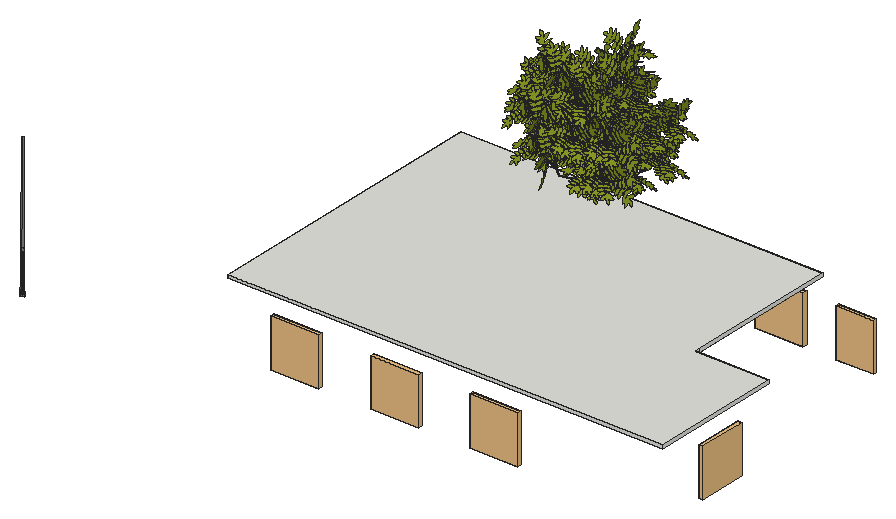
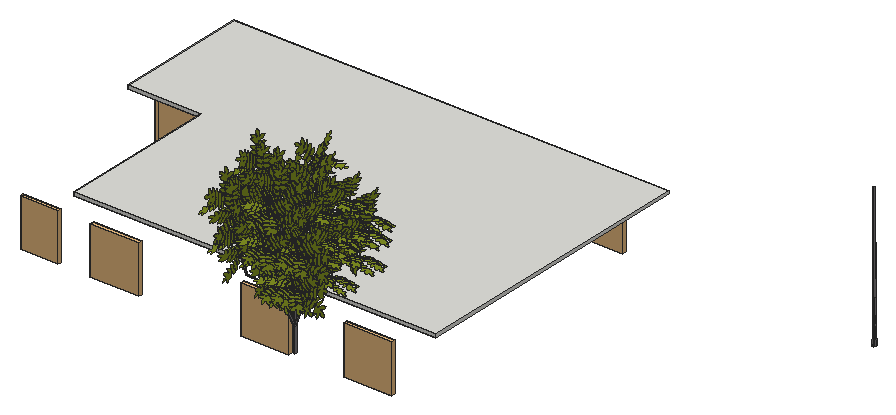
# SketchUp Ruby script. Lengths in inches.
U = 1.inch
M = Sketchup.active_model
def pt(a) = Geom::Point3d.new(a.map { |v| v * U })
def face(e, loops, mat)
  f = e.add_face(loops[0].map { |a| pt(a) })
  loops[1..].each { |l| e.add_face(l.map { |a| pt(a) }).erase! }
  f.material = f.back_material = mat if mat
  f
end
# faces: each face lists its corners as indices into pts; further lists are holes
def faces(e, pts, list, mat = nil) = list.each { |f| face(e, (f[0].is_a?(Array) ? f : [f]).map { |l| l.map { |i| pts[i] } }, mat) }
# xy, xz, yz: faces in a plane at the given z, y or x. An outline is a flat list of corners, or four numbers for a rectangle; further outlines are holes
def ring(l) = l.size == 4 ? [[l[0], l[1]], [l[2], l[1]], [l[2], l[3]], [l[0], l[3]]] : l.each_slice(2).to_a
def flat(e, list, mat, &to3) = list.each { |f| face(e, (f[0].is_a?(Array) ? f : [f]).map { |l| ring(l).map { |u, v| to3.(u, v) } }, mat) }
def xy(e, z, list, mat = nil) = flat(e, list, mat) { |x, y| [x, y, z] }
def xz(e, y, list, mat = nil) = flat(e, list, mat) { |x, z| [x, y, z] }
def yz(e, x, list, mat = nil) = flat(e, list, mat) { |y, z| [x, y, z] }
def lines(e, pts, list) = list.each { |a, b| e.add_line(pt(pts[a]), pt(pts[b])) }
# prism: a flat outline (further loops are holes) pulled along v
def prism(e, loops, v, mat = nil)
  f = face(e, loops, mat); d = Geom::Vector3d.new(v.map { |x| x * U })
  f.pushpull(f.normal.samedirection?(d) ? d.length : -d.length)
end
def box(e, o, s, mat = nil) = prism(e, [[o, [o[0] + s[0], o[1], o[2]], [o[0] + s[0], o[1] + s[1], o[2]], [o[0], o[1] + s[1], o[2]]]], [0, 0, s[2]], mat)
def at(x, y, z, deg = 0) = Geom::Transformation.translation(pt([x, y, z])) * Geom::Transformation.rotation(ORIGIN, Z_AXIS, deg.degrees)
def axes(o, x, y, z) = Geom::Transformation.new([*x, 0, *y, 0, *z, 0, *pt(o).to_a, 1])
def part(name) = M.definitions.add(name)
# library, detail: a bought-in or finely detailed component or shape, given as its bounding box
def library(name, o, s) = part(name).tap { |d| box(d.entities, o, s) }
def detail(e, o, s) = box(e.add_group.entities, o, s)
def put(e, d, t, mat = nil) = e.add_instance(d, t).tap { |i| i.material = mat if mat }
def group(e, t, mat = nil) = e.add_group.tap { |g| g.transformation = t; g.material = mat if mat }.entities
root = M.entities
M.materials.add("3D66_SU_1574822641685_001").color = [135, 150, 36]
M.materials.add("3D66_SU_1574822641883_002").color = [178, 165, 164]
M.materials.add("3D66_SU_1574822642012_003").color = [128, 125, 127]
c1 = library("4e1fe49e-2fec-46be-a265-c81cc17eb477",[0,0,0],[35.43,4.93,59.06])
c2 = part("rama-acacia")
p = [[-13.8,1.01,-1.08],[-13.61,0.91,-1.04],[-13.61,0.85,-1.06],[-14.07,0.85,-1.21],[-15.17,0.86,-1.58],[-15.95,0.92,-1.83],
  [-16.01,1,-1.83],[-16.01,1.17,-1.78],[-16.07,1.93,-1.6],[-16.4,2.73,-1.5],[-16.65,3.06,-1.5],[-17.13,4.01,-1.41],
  [-17.78,4.7,-1.44],[-18.28,5.07,-1.51],[-18.57,5.18,-1.58],[-18.91,5.47,-1.62],[-19.07,5.48,-1.67],[-19.35,5.61,-1.73],
  [-19.51,5.64,-1.78],[-19.38,5.57,-1.75],[-19.33,5.5,-1.75],[-19.31,5.23,-1.82],[-19.38,5.08,-1.89],[-19.41,4.84,-1.96],
  [-19.36,4.59,-2.01],[-19.43,4.55,-2.04],[-19.36,4.15,-2.125],[-19.21,3.7,-2.19],[-18.875,3.1,-2.24],[-18.61,2.78,-2.24],
  [-17.83,2.19,-2.13],[-17.4375,1.85,-2.09],[-17.04,1.49,-2.05],[-16.61,1.24,-1.97],[-16.17,1.0625,-1.87],[-16.06,0.95,-1.86],
  [-16.06,0.91,-1.87],[-16.32,0.9,-1.96],[-16.7,0.88,-2.1],[-17.05,0.91,-2.21],[-17.61,1.15,-2.33],[-18.06,1.29,-2.45],
  [-18.88,1.53,-2.67],[-20.25,1.46,-3.15],[-20.59,1.49,-3.26],[-20.79,1.37,-3.36],[-21.08,1.2,-3.5],[-21.28,1.22,-3.5625],
  [-21.48,0.94,-3.71],[-21.79,0.5,-3.93],[-22.02,0.17,-4.1],[-22.11,0.05,-4.16],[-22.21,-0.02,-4.21],[-22.375,-0.05,-4.28],
  [-22.375,-0.07,-4.28],[-22.18,-0.09,-4.22],[-22.11,-0.07,-4.19],[-21.78,-0.1,-4.09],[-21.6,-0.18,-4.05],[-21.52,-0.27,-4.04],
  [-21.33,-0.33,-4],[-20.94,-0.54,-3.92],[-20.6875,-0.63,-3.86],[-20.54,-0.68,-3.82],[-20.42,-0.67,-3.78],[-20.09,-0.46,-3.61],
  [-19.8,-0.24,-3.45],[-19.21,-0.02,-3.19],[-18.48,0.08,-2.92],[-17.72,0.38,-2.58],[-17.4,0.5,-2.4375],[-16.93,0.75,-2.21],
  [-16.78,0.8,-2.15],[-16.1,0.83,-1.91],[-16.0625,0.81,-1.9],[-16.08,0.77,-1.91],[-16.27,0.72,-1.99],[-16.88,0.39,-2.29],
  [-17.1875,0.15,-2.46],[-17.27,0.02,-2.52],[-17.94,-0.52,-2.89],[-17.94,-0.59,-2.91],[-18.08,-0.68,-2.99],[-18.13,-0.86,-3.05],
  [-18.56,-1.55,-3.38],[-18.71,-2.11,-3.58],[-18.79,-2.61,-3.74],[-18.86,-2.84,-3.83],[-18.87,-3.07,-3.89],[-18.84,-3.22,-3.92],
  [-18.8,-3.26,-3.92],[-18.76,-3.47,-3.96],[-18.76,-3.6,-4],[-18.67,-3.8,-4.02],[-18.61,-3.92,-4.04],[-18.58,-4.11,-4.07],
  [-18.53,-4.18,-4.08],[-18.58,-4.35,-4.14],[-18.65,-4.43,-4.18],[-18.72,-4.51,-4.23],[-18.8125,-4.51,-4.26],[-18.8125,-4.53,-4.26],
  [-18.72,-4.54,-4.24],[-18.66,-4.49,-4.21],[-18.58,-4.43,-4.16],[-18.35,-4.23,-4.03],[-18.32,-4.17,-4],[-18.22,-4.125,-3.95],
  [-18.1,-4,-3.88],[-17.79,-3.72,-3.7],[-17.68,-3.51,-3.61],[-17.32,-3.13,-3.38],[-17.24,-2.94,-3.31],[-16.78,-2.12,-2.93],
  [-16.48,-1.78,-2.73],[-16.3,-1.28,-2.54],[-16.05,-0.75,-2.3125],[-15.89,-0.2,-2.11],[-15.89,0.39,-1.95],[-15.96,0.79,-1.87],
  [-15.91,0.82,-1.84],[-15.27,0.8,-1.63],[-14.18,0.76,-1.27],[-13.78,0.73,-1.15],[-13.78,0.67,-1.16],[-14.23,0.54,-1.35],
  [-14.65,0.33,-1.55],[-14.97,0.02,-1.74],[-15.25,-0.36,-1.9375],[-15.57,-0.72,-2.14],[-15.96,-1.64,-2.52],[-16.2,-2.51,-2.84],
  [-16.2,-3.12,-3],[-16.14,-3.41,-3.06],[-16.1,-3.75,-3.14],[-16.1,-4.09,-3.23],[-16.2,-4.25,-3.3],[-16.2,-4.28,-3.3125],
  [-16.08,-4.19,-3.24],[-15.98,-4.08,-3.18],[-15.96,-3.94,-3.14],[-15.96,-3.8125,-3.1],[-15.9,-3.72,-3.06],[-15.68,-3.55,-2.9375],
  [-15.51,-3.49,-2.86],[-15.3,-3.33,-2.75],[-15.23,-3.17,-2.68],[-15.01,-3.03,-2.57],[-14.875,-2.83,-2.47],[-14.6,-2.59,-2.3125],
  [-14.4,-2.27,-2.16],[-14.12,-1.6,-1.89],[-13.91,-1.1,-1.68],[-13.67,-0.83,-1.53],[-13.53,-0.45,-1.38],[-13.53,0.67,-1.08],
  [-13.53,0.69,-1.07],[-13.38,0.86,-0.98],[-13.38,0.92,-0.96],[-13.32,1.03,-0.91],[-13.32,1.35,-0.82],[-13.28,1.49,-0.77],
  [-13.28,1.99,-0.64],[-13.44,2.67,-0.51],[-13.72,3.31,-0.43],[-13.93,3.71,-0.4],[-14.1,4.39,-0.27],[-14.5625,5.06,-0.25],
  [-14.89,5.62,-0.21],[-15.33,6.1,-0.23],[-15.65,6.8,-0.15],[-15.79,6.89,-0.18],[-15.61,6.52,-0.22],[-15.51,6.32,-0.24],
  [-15.45,6.28,-0.23],[-15.52,6,-0.32],[-15.63,5.6875,-0.45],[-15.77,4.97,-0.68],[-15.7,4.25,-0.85],[-15.46,3,-1.11],
  [-15,2.03,-1.21],[-14.3,1.29,-1.17],[-12.41,6.01,0.65],[-12.44,6.14,0.68],[-12.41,6.29,0.73],[-12.43,6.29,0.73],
  [-12.44,6.26,0.72],[-12.47,6.15,0.68],[-12.49,6.07,0.66],[-12.57,5.75,0.55],[-12.67,5.36,0.43],[-12.79,4.875,0.28],
  [-12.83,4.52,0.18],[-12.83,3.99,0.04],[-12.73,3.11,-0.18],[-12.58,2.52,-0.3125],[-12.3,1.97,-0.41],[-11.88,1.51,-0.46],
  [-11.37,1.0625,-0.48],[-10.75,0.75,-0.45],[-10.75,0.68,-0.47],[-12.55,0.7,-0.79],[-13.21,0.79,-0.89],[-13.2,0.67,-0.92],
  [-12.56,0.62,-0.82],[-11.15,0.56,-0.58],[-10.79,0.54,-0.52],[-10.72,0.52,-0.51],[-10.72,0.5,-0.52],[-10.87,0.47,-0.55],
  [-11.14,0.41,-0.62],[-11.39,0.27,-0.7],[-11.625,-0.01,-0.82],[-11.8,-0.43,-0.96],[-11.83,-0.57,-1],[-12.02,-1.08,-1.17],
  [-12.1,-1.39,-1.27],[-12.17,-1.95,-1.4375],[-12.17,-2.77,-1.65],[-12.09,-3.59,-1.86],[-11.86,-4.26,-2],[-11.8125,-4.4,-2.03],
  [-11.84,-4.49,-2.05],[-11.91,-4.6,-2.1],[-11.97,-4.65,-2.12],[-11.98,-4.67,-2.13],[-11.92,-4.65,-2.11],[-11.84,-4.59,-2.08],
  [-11.77,-4.52,-2.05],[-11.74,-4.47,-2.03],[-11.37,-4.3125,-1.92],[-10.95,-4.0625,-1.78],[-10.82,-3.89,-1.71],[-10.64,-3.57,-1.59],
  [-10.41,-3.05,-1.41],[-10.27,-2.73,-1.3],[-10.07,-1.88,-1.03],[-10.15,-0.71,-0.73],[-10.31,-0.1,-0.6],[-10.5,0.4,-0.5],
  [-10.5,0.48,-0.48],[-10.44,0.53,-0.45],[-10.39,0.64,-0.42],[-10.52,0.73,-0.42],[-10.44,0.93,-0.35],[-10.44,1.2,-0.28],
  [-10.32,1.47,-0.18],[-10.48,2.6875,0.12],[-10.43,2.96,0.2],[-10.75,3.87,0.38],[-11.26,4.93,0.57],[-11.8,5.54,0.64],
  [-12.37,5.93,0.64],[-7.78,0.19,-0.06],[-7.78,0.25,-0.04],[-7.75,0.39,0],[-7.89,0.4,-0.02],[-7.96,0.46,-0.02],
  [-7.96,0.49,-0.01],[-7.76,0.62,0.06],[-7.53,0.99,0.2],[-7.31,1.78,0.45],[-7.31,2.74,0.71],[-7.63,3.6875,0.9],
  [-8.02,4.57,1.07],[-8.66,5.23,1.13],[-8.83,5.4,1.14],[-8.92,5.54,1.16],[-9.1,5.64,1.16],[-9.08,5.6,1.15],
  [-9.02,5.56,1.15],[-8.94,5.46,1.14],[-8.9,5.37,1.12],[-8.9375,5.25,1.08],[-9.14,4.92,0.96],[-9.31,4.5625,0.83],
  [-9.39,3.73,0.6],[-9.44,2.76,0.32],[-9.23,1.59,0.05],[-8.82,0.9,-0.06],[-8.36,0.59,-0.0625],[-8.14,0.51,-0.04],
  [-8.05,0.48,-0.03],[-8.05,0.46,-0.04],[-8.12,0.43,-0.06],[-10.1,0.49,-0.4],[-8.22,0.3125,-0.11],[-8.22,0.25,-0.125],
  [-8.53,0.13,-0.21],[-8.8,-0.16,-0.34],[-8.96,-0.61,-0.49],[-8.96,-0.87,-0.56],[-9.16,-1.42,-0.74],[-9.13,-1.77,-0.83],
  [-9.09,-1.83,-0.84],[-9.125,-1.92,-0.87],[-9.125,-2.13,-0.93],[-9.08,-2.23,-0.95],[-9.15,-2.39,-1],[-9.11,-2.67,-1.07],
  [-9.03,-2.86,-1.11],[-9.07,-3.03,-1.16],[-8.97,-3.23,-1.19],[-8.93,-3.44,-1.24],[-8.93,-3.71,-1.32],[-8.79,-4.05,-1.38],
  [-8.7,-4.25,-1.42],[-8.7,-4.39,-1.46],[-8.76,-4.53,-1.5],[-8.77,-4.65,-1.54],[-8.64,-4.55,-1.49],[-8.27,-4.22,-1.33],
  [-8.1875,-4.06,-1.27],[-8.07,-3.98,-1.23],[-7.98,-3.79,-1.17],[-7.79,-3.59,-1.08],[-7.64,-3.3,-0.97],[-7.64,-3.25,-0.96],
  [-7.59,-3.21,-0.9375],[-7.52,-2.93,-0.85],[-7.52,-2.85,-0.83],[-7.47,-2.81,-0.81],[-7.3,-2.09,-0.59],[-7.32,-2.01,-0.57],
  [-7.27,-1.95,-0.54],[-7.1875,-1.57,-0.42],[-7.17,-1.46,-0.39],[-7.17,-1.16,-0.3125],[-7.23,-0.61,-0.17],[-7.49,-0.15,-0.1],
  [-13.39,-0.07,-1.23],[-13.39,0.25,-1.14],[-13.49,0.5625,-1.09],[-4.5625,0.33,0.09],[-4.22,0.49,0.13],[-4,0.7,0.1875],
  [-3.86,0.99,0.26],[-3.77,1.41,0.38],[-3.7,1.73,0.46],[-3.77,1.99,0.53],[-3.85,2.17,0.58],[-3.88,2.57,0.6875],
  [-3.98,2.9,0.78],[-4.0625,2.97,0.8],[-4.1,3.14,0.84],[-4.1875,3.25,0.87],[-4.27,3.55,0.95],[-4.31,3.71,0.99],
  [-4.42,3.9,1.04],[-4.625,4.2,1.125],[-4.72,4.39,1.18],[-4.89,4.57,1.23],[-4.98,4.73,1.27],[-5,4.72,1.26],
  [-5.01,4.51,1.21],[-4.96,4.32,1.16],[-4.97,4.27,1.14],[-5.14,3.78,1.01],[-5.3,3.39,0.91],[-5.44,2.76,0.74],
  [-5.5,2.09,0.56],[-5.57,1.78,0.48],[-5.57,1.42,0.38],[-5.57,1.09,0.29],[-5.47,0.72,0.19],[-5.22,0.44,0.12],
  [-4.93,0.27,0.07],[-4.76,0.22,0.06],[-4.76,0.18,0.05],[-4.83,0.16,0.04],[-5.26,0,0],[-5.34,-0.04,-0.01],
  [-5.47,-0.22,-0.06],[-5.51,-0.6,-0.16],[-5.42,-1.09,-0.29],[-5.28,-1.49,-0.4],[-5.21,-1.87,-0.5],[-5.11,-2.15,-0.57],
  [-5.08,-2.34,-0.63],[-5.01,-2.47,-0.66],[-4.96,-2.69,-0.72],[-4.86,-2.9375,-0.79],[-4.84,-3.07,-0.82],[-4.77,-3.18,-0.85],
  [-4.74,-3.43,-0.92],[-4.7,-3.71,-0.99],[-4.62,-3.89,-1.04],[-4.58,-3.98,-1.07],[-4.58,-3.83,-1.03],[-4.51,-3.67,-0.98],
  [-4.3,-3.32,-0.89],[-4.16,-3.09,-0.83],[-4.16,-2.98,-0.8],[-4.11,-2.92,-0.78],[-4.02,-2.8,-0.75],[-3.95,-2.59,-0.69],
  [-3.95,-2.33,-0.625],[-3.86,-2.26,-0.6],[-3.86,-2.02,-0.54],[-3.86,-1.44,-0.39],[-3.94,-1.22,-0.33],[-3.94,-1.08,-0.29],
  [-4,-0.96,-0.26],[-4,-0.87,-0.23],[-4.0625,-0.8125,-0.22],[-4.16,-0.54,-0.14],[-4.39,-0.24,-0.06],[-4.61,-0.08,-0.02],
  [-4.77,-0.03,-0.01],[-4.77,-0.01,0],[-4.65,-0.01,0],[-4.61,0.19,0.05],[-4.66,0.23,0.0625],[-4.63,0.29,0.08],
  [-4.07,0.17,0.04],[0,-0.24,-0.06],[0,0,0],[-0.5,0.04,0.01],[-1.58,0.08,0.02]]
faces(c2.entities,p,[[0,1,2,3,4,5,6,7,8,9,10,11,12,13,14,15,16,17,18,19,20,21,22,23,24,25,26,27,28,29,30,31,32,33,34,35,36,37,38,39,40,41,42,43,44,45,46,47,48,49,50,51,52,53,54,55,56,57,58,59,60,61,62,63,64,65,66,67,68,69,70,71,72,73,74,75,76,77,78,79,80,81,82,83,84,85,86,87,88,89,90,91,92,93,94,95,96,97,98,99,100,101,102,103,104,105,106,107,108,109,110,111,112,113,114,115,116,117,118,119,120,121,122,123,124,125,126,127,128,129,130,131,132,133,134,135,136,137,138,139,140,141,142,143,144,145,146,147,148,149,150,151,152,153,154,155,156,157,158,159,160,161,162,163,164,165,166,167,168,169,170,171,172,173,174,175,176,177,178,179,180,181],[182,183,184,185,186,187,188,189,190,191,192,193,194,195,196,197,198,199,200,201,202,203,204,205,206,207,208,209,210,211,212,213,214,215,216,217,218,219,220,221,222,223,224,225,226,227,228,229,230,231,232,233,234,235,236,237,238,239,240,241,242,243,244,245,246,247,248,249,250,251,252],[253,254,255,256,257,258,259,260,261,262,263,264,265,266,267,268,269,270,271,272,273,274,275,276,277,278,279,280,281,282,283,284,242,241,285,286,287,288,289,290,291,292,293,294,295,296,297,298,299,300,301,302,303,304,305,306,307,308,309,310,311,312,313,314,315,316,317,318,319,320,321,322,323,324,325,326,327,328,329],[154,330,331,332,155],[333,334,335,336,337,338,339,340,341,342,343,344,345,346,347,348,349,350,351,352,353,354,355,356,357,358,359,360,361,362,363,364,365,366,367,368,369,370,371,372,373,374,375,376,377,378,379,380,381,382,383,384,385,386,387,388,389,390,391,392,393,394,395,396,397,398,399,400,401,402,403,404,405,406,407,408,409,410,411,412,413],[156,203,157],[202,157,203],[414,411,410,415,416,417,418],
  [254,370,255],[369,255,370]],"3D66_SU_1574822641685_001")
c3 = part("ramas")
put(c3.entities,c2,axes([0.11,0.06,-0.22],[-0.42655,-0.79206,-0.43668],[0.22445,0.37501,-0.89944],[0.87617,-0.48167,0.01782]))
put(c3.entities,c2,axes([0.14,0.21,0.02],[0.24321,-0.08852,-0.96593],[0.34202,0.93969,0],[0.90767,-0.33037,0.25882]))
put(c3.entities,c2,at(0,0.24,0.06))
put(c3.entities,c2,axes([0.11,0.45,0.57],[-0.42655,0.68302,0.5929],[0.22445,-0.55509,0.80093],[0.87617,0.47472,0.08347]))
put(c3.entities,c2,axes([0.11,0.73,0.01],[-0.42655,0.88928,-0.16503],[0.22445,0.28083,0.93314],[0.87617,0.36099,-0.31939]))
c4 = part("rama principal")
put(c4.entities,c2,axes([-20.25,-0.15,12.84],[0.38818,-0.89018,-0.23852],[0.89018,0.42916,-0.15296],[0.23852,-0.15296,0.95902]))
put(c4.entities,c2,at(-20.48,0,12.88))
put(c4.entities,c2,axes([-20.6875,-0.1,12.85],[0.57358,0.79124,0.21201],[-0.79124,0.60214,-0.10661],[-0.21201,-0.10661,0.97144]))
put(c4.entities,c2,axes([-20.375,-0.01,13.02],[-0.37792,0.77975,-0.49916],[-0.65887,0.15226,0.73669],[0.65043,0.60729,0.45621]))
put(c4.entities,c2,axes([-20.34,-0.04,12.83],[0.24321,-0.08852,-0.96593],[0.34202,0.93969,0],[0.90767,-0.33037,0.25882]))
put(c4.entities,c2,axes([-20.375,-0.18,12.6],[-0.42655,-0.79206,-0.43668],[0.22445,0.37501,-0.89944],[0.87617,-0.48167,0.01782]))
put(c4.entities,c3,at(-11.43,0,7.77))
g1 = group(c4.entities,at(0,0.2,0),"3D66_SU_1574822641883_002")
xz(g1,0.1,[[-0.15,-0.08,-3.26,5.59,-11.5,7.61,-18.23,12.71,-20.48,12.71,-20.48,13.05,-18.11,13.05,-11.35,7.92,-3.03,5.89,0.15,0.08]])
yz(g1,-20.48,[[0.1,12.71,-0.2,12.88,0.1,13.05]])
p = [[-0.15,0.1,-0.08],[0,-0.2,0],[-3.15,-0.2,5.74],[-3.26,0.1,5.59],[0.15,0.1,0.08],[-3.03,0.1,5.89],
  [-11.43,-0.2,7.77],[-11.5,0.1,7.61],[-11.35,0.1,7.92],[-18.17,-0.2,12.88],[-18.23,0.1,12.71],[-18.11,0.1,13.05],
  [-20.48,-0.2,12.88],[-20.48,0.1,12.71],[-20.48,0.1,13.05]]
faces(g1,p,[[0,1,2,3],[0,4,1],[1,4,5,2],[3,2,6,7],[2,5,8,6],[7,6,9,10],[6,8,11,9],[10,9,12,13],
  [9,11,14,12]])
c5 = part("Component\#1")
p = [[44.23,0.79,16.51],[35.57,0.79,41.625],[19.17,0.79,51.61],[7.37,0.79,32.7],[0.16,0.79,57.85],[31.31,0.79,23.98]]
lines(c5.entities,p,[[0,1],[1,2],[3,4],[5,3]])
g2 = group(c5.entities,at(44.23,0.79,-28.39))
xz(g2,0.2,[[-0.32,44.79,-8.95,69.78,-25.24,79.7,-24.89,80.28,-8.38,70.24,0.32,45.01]],"3D66_SU_1574822642012_003")
p = [[-0.32,0.2,44.79],[0,-0.39,44.9],[-8.67,-0.39,70.01],[-8.95,0.2,69.78],[0.32,0.2,45.01],[-8.38,0.2,70.24],
  [-25.06,-0.39,79.99],[-25.24,0.2,79.7],[-24.89,0.2,80.28]]
faces(g2,p,[[0,1,2,3],[0,4,1],[1,4,5,2],[3,2,6,7],[2,5,8,6],[8,7,6]],"3D66_SU_1574822642012_003")
g3 = group(c5.entities,at(44.23,0.79,-28.39),"3D66_SU_1574822642012_003")
p = [[-0.6,0.39,28.39],[0,-0.79,28.71],[-12.89,-0.52,52.37],[-13.25,0.19,52.17],[0.6,0.39,29.04],[-12.53,0.19,52.57]]
faces(g3,p,[[0,1,2,3],[4,0,3,5],[1,4,5,2]],"3D66_SU_1574822642012_003")
faces(g3,p,[[0,4,1],[5,3,2]])
g4 = group(c5.entities,at(44.23,0.79,-28.39))
prism(g4,[[[-37.03,0.1,61.04],[-36.7,0.1,61.13],[-36.86,-0.2,61.08]]],[-7.21,0,25.15],"3D66_SU_1574822642012_003")
g5 = group(c5.entities,at(44.23,0.79,-28.39))
prism(g5,[[[-13.04,0.2,52.05],[-12.81,0.2,52.69],[-12.92,-0.39,52.37]]],[-23.94,0,8.71],"3D66_SU_1574822642012_003")
c6 = part("Group\#7")
p = [[74.89,60.42,11.53],[61.97,60.42,35.1875]]
lines(c6.entities,p,[[0,1]])
put(c6.entities,c4,at(68.97,49.02,23.76))
put(c6.entities,c4,at(53.09,47.85,77.85))
put(c6.entities,c4,at(71.03,52.76,41.54))
put(c6.entities,c5,at(57.21,20.01,0,65))
put(c6.entities,c5,at(36.98,37.62,26.03,30))
put(c6.entities,c4,at(64.15,37.99,51.46))
put(c6.entities,c4,at(56.21,20.74,57.94))
put(c6.entities,c4,at(58.92,27.24,32.75))
put(c6.entities,c4,at(63.69,53.97,50.16))
put(c6.entities,c4,at(67.38,56.1,67.8))
put(c6.entities,c4,at(42.86,42.51,58.92))
p = [[862.87,278.08,118],[871.06,278.08,118]]
lines(root,p,[[0,1]])
g6 = group(root,at(98.11,92.93,-24.1))
xy(g6,48.23,[[-1.25,-1.68,-1.25,1.85,2.29,0.08]])
xy(g6,102.61,[[-0.6,-1.2,1.63,0,-0.6,1.2]])
p = [[-1.25,1.85,48.23],[-1.25,-1.68,48.23],[-0.6,1.2,102.61],[2.29,0.08,48.23],[2.0625,0,61.83],[-1.03,-1.66,61.83],
  [-1.03,1.66,61.83],[-1.03,1.66,75.42],[2.0625,0,75.42],[-1.03,-1.66,75.42],[1.63,0,102.61],[-0.6,-1.2,102.61]]
faces(g6,p,[[0,1,2],[3,4,1],[1,4,5],[1,5,2],[4,3,6],[0,6,3],[2,0,7],[6,7,0],
  [4,8,9,5],[9,2,5],[6,7,8,4],[8,10,11,9],[11,2,9],[7,2,10,8]],"3D66_SU_1574822642012_003")
put(root,c1,axes([867.12,233.8125,35.43],[0,-1.68604,0],[1,0,0],[0,0,1]))
put(root,c1,axes([632.85,113.59,35.43],[1.68604,0,0],[0,1,0],[0,0,1]))
put(root,c1,axes([510.89,113.59,35.43],[1.68604,0,0],[0,1,0],[0,0,1]))
put(root,c1,axes([387.34,113.59,35.43],[1.68604,0,0],[0,1,0],[0,0,1]))
put(root,c1,axes([800.21,469.65,35.43],[1.31071,0,0],[0,0.79898,0],[0,0,1]))
put(root,c1,axes([514.73,469.65,35.43],[1.68604,0,0],[0,1,0],[0,0,1]))
put(root,c1,axes([387.73,469.65,35.43],[1.68604,0,0],[0,1,0],[0,0,1]))
put(root,c1,axes([699.88,469.65,35.43],[1.68604,0,0],[0,1,0],[0,0,1]))
g7 = group(root,at(496.38,488.14,50.32),"3D66_SU_1574822642012_003")
xy(g7,0,[[-1.29,-2.08,-1.29,2.08,2.58,0]])
xy(g7,48.23,[[-1.02,-1.79,2.31,0,-1.02,1.79]])
p = [[2.58,0,0],[2.31,0,48.23],[-1.02,-1.79,48.23],[-1.29,-2.08,0],[-1.02,1.79,48.23],[-1.29,2.08,0]]
faces(g7,p,[[0,1,2,3],[2,4,5,3],[5,4,1,0]])
g8 = group(root,at(98.42,92.96,-24.1))
xy(g8,102.61,[[-0.92,-1.17,-0.92,1.17,1.3125,0]],"3D66_SU_1574822642012_003")
xy(g8,224.33,[[-0.4,-0.625,0.79,0,-0.4,0.625]],"3D66_SU_1574822642012_003")
p = [[-0.4,-0.625,224.33],[-0.4,0.625,224.33],[-0.92,1.17,102.61],[-0.92,-1.17,102.61],[1.3125,0,102.61],[0.79,0,224.33]]
faces(g8,p,[[0,1,2,3],[4,5,0,3],[2,1,5,4]],"3D66_SU_1574822642012_003")
put(root,c6,axes([429.02,587.37,79.18],[-0.15043,-1.21193,0],[1.30133,-0.1401,0],[0,0,1.6799]))
put(root,c6,axes([398.27,414.44,79.18],[1.31,0,0],[0,1.22,0],[0,0,1.6799]))
put(root,c6,axes([620.92,506.29,79.18],[-1.13449,0.61,0],[-0.655,-1.05655,0],[0,0,1.6799]))
put(root,c6,axes([566.68,390.7,79.18],[0.11417,1.21536,0],[-1.30502,0.10633,0],[0,0,1.6799]))
g9 = group(root,at(496.38,488.14,50.32))
xy(g9,48.23,[[-1.25,-1.68,-1.25,1.85,2.29,0.08]])
xy(g9,102.61,[[-0.6,-1.2,1.63,0,-0.6,1.2]])
p = [[-1.25,1.85,48.23],[-1.25,-1.68,48.23],[-0.6,1.2,102.61],[2.29,0.08,48.23],[2.0625,0,61.83],[-1.03,-1.66,61.83],
  [-1.03,1.66,61.83],[-1.03,1.66,75.42],[2.0625,0,75.42],[-1.03,-1.66,75.42],[1.63,0,102.61],[-0.6,-1.2,102.61]]
faces(g9,p,[[0,1,2],[3,4,1],[1,4,5],[1,5,2],[4,3,6],[0,6,3],[2,0,7],[6,7,0],
  [4,8,9,5],[9,2,5],[6,7,8,4],[8,10,11,9],[11,2,9],[7,2,10,8]],"3D66_SU_1574822642012_003")
g10 = group(root,at(334.375,113.59,118))
xy(g10,0,[[0,0,0,360,446.44,360,446.44,163.875,536.68,163.875,536.68,0]])
xy(g10,3.94,[[0,0,536.68,0,536.68,163.875,446.44,163.875,446.44,360,0,360]])
xz(g10,0,[[0,0,536.68,3.94]])
xz(g10,163.875,[[446.44,0,536.68,3.94]])
xz(g10,360,[[0,0,446.44,3.94]])
yz(g10,0,[[0,0,360,3.94]])
yz(g10,446.44,[[163.875,0,168.8125,3.94],[168.8125,0,360,3.94]])
yz(g10,536.68,[[0,0,163.875,3.94]])
p = [[446.44,359.22,0],[451.25,359.22,0]]
lines(g10,p,[[0,1]])
